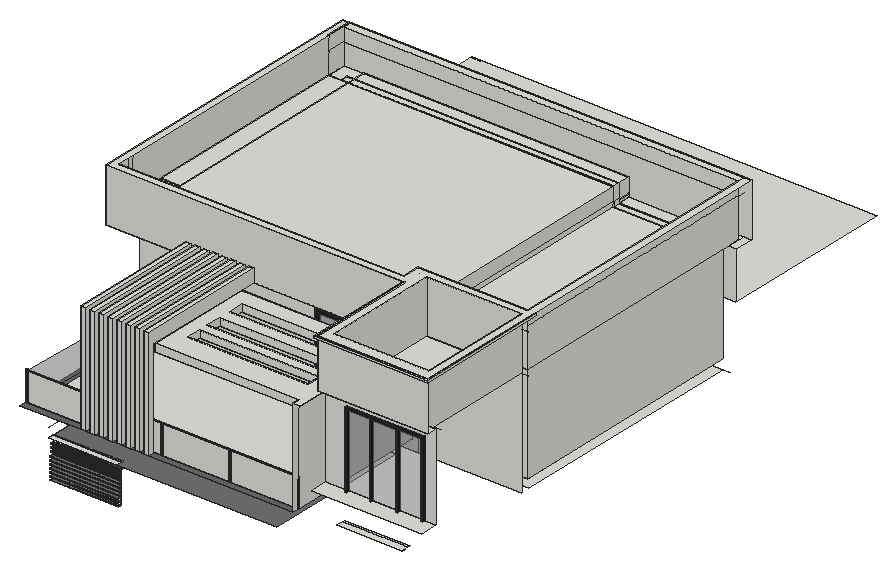
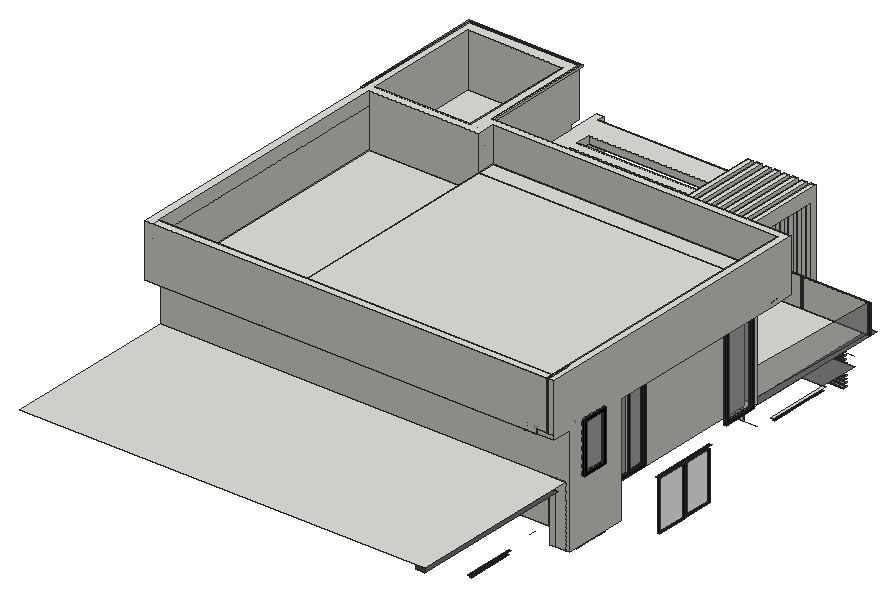
# SketchUp Ruby script. Lengths in inches.
U = 1.inch
M = Sketchup.active_model
def pt(a) = Geom::Point3d.new(a.map { |v| v * U })
def face(e, loops, mat)
  f = e.add_face(loops[0].map { |a| pt(a) })
  loops[1..].each { |l| e.add_face(l.map { |a| pt(a) }).erase! }
  f.material = f.back_material = mat if mat
  f
end
# faces: each face lists its corners as indices into pts; further lists are holes
def faces(e, pts, list, mat = nil) = list.each { |f| face(e, (f[0].is_a?(Array) ? f : [f]).map { |l| l.map { |i| pts[i] } }, mat) }
# xy, xz, yz: faces in a plane at the given z, y or x. An outline is a flat list of corners, or four numbers for a rectangle; further outlines are holes
def ring(l) = l.size == 4 ? [[l[0], l[1]], [l[2], l[1]], [l[2], l[3]], [l[0], l[3]]] : l.each_slice(2).to_a
def flat(e, list, mat, &to3) = list.each { |f| face(e, (f[0].is_a?(Array) ? f : [f]).map { |l| ring(l).map { |u, v| to3.(u, v) } }, mat) }
def xy(e, z, list, mat = nil) = flat(e, list, mat) { |x, y| [x, y, z] }
def xz(e, y, list, mat = nil) = flat(e, list, mat) { |x, z| [x, y, z] }
def yz(e, x, list, mat = nil) = flat(e, list, mat) { |y, z| [x, y, z] }
def lines(e, pts, list) = list.each { |a, b| e.add_line(pt(pts[a]), pt(pts[b])) }
# prism: a flat outline (further loops are holes) pulled along v
def prism(e, loops, v, mat = nil)
  f = face(e, loops, mat); d = Geom::Vector3d.new(v.map { |x| x * U })
  f.pushpull(f.normal.samedirection?(d) ? d.length : -d.length)
end
def box(e, o, s, mat = nil) = prism(e, [[o, [o[0] + s[0], o[1], o[2]], [o[0] + s[0], o[1] + s[1], o[2]], [o[0], o[1] + s[1], o[2]]]], [0, 0, s[2]], mat)
def at(x, y, z, deg = 0) = Geom::Transformation.translation(pt([x, y, z])) * Geom::Transformation.rotation(ORIGIN, Z_AXIS, deg.degrees)
def axes(o, x, y, z) = Geom::Transformation.new([*x, 0, *y, 0, *z, 0, *pt(o).to_a, 1])
def part(name) = M.definitions.add(name)
# library, detail: a bought-in or finely detailed component or shape, given as its bounding box
def library(name, o, s) = part(name).tap { |d| box(d.entities, o, s) }
def detail(e, o, s) = box(e.add_group.entities, o, s)
def put(e, d, t, mat = nil) = e.add_instance(d, t).tap { |i| i.material = mat if mat }
def group(e, t, mat = nil) = e.add_group.tap { |g| g.transformation = t; g.material = mat if mat }.entities
root = M.entities
M.materials.add("[0134_DimGray]").color = [105, 105, 105]
M.materials.add("[0136_Charcoal]").color = [35, 35, 35]
M.materials.add("[0137_Black]").color = [0, 0, 0]
M.materials.add("[Color M05]").color = [114, 114, 114]
M.materials.add("[Color M06]").color = [86, 86, 86]
M.materials.add("[Color M08]").color = [30, 30, 30]
M.materials.add("[Marble Carrara Gold Floor Tile]").color = [225, 223, 217]
M.materials.add("[Translucent Glass Gray]").color = [128, 128, 128]
M.materials["[Translucent Glass Gray]"].alpha = 0.5
c1 = part("Group\#89")
box(c1.entities,[-152.36,0,0],[152.36,1.57,1.57])
c2 = part("Glass+Wall")
g1 = group(c2.entities,at(79.73,0,0))
g2 = group(g1,at(0,0,0))
g3 = group(g2,at(195.28,0,0),"[0136_Charcoal]")
box(g3,[-195.28,0,0],[195.28,1.57,1.57])
put(g2,c1,axes([1.57,0,116.54],[0,0,0.75452],[0,1,0],[-1,0,0]),"[0136_Charcoal]")
put(g2,c1,axes([50,0,116.54],[0,0,0.75452],[0,1,0],[-1,0,0]),"[0136_Charcoal]")
g4 = group(g2,at(195.28,0,115.75),"[0136_Charcoal]")
box(g4,[-195.28,0,0.79],[195.28,1.57,1.57])
put(g2,c1,axes([98.43,0,116.54],[0,0,0.75452],[0,1,0],[-1,0,0]),"[0136_Charcoal]")
put(g2,c1,axes([146.85,0,116.54],[0,0,0.75452],[0,1,0],[-1,0,0]),"[0136_Charcoal]")
put(g2,c1,axes([195.28,0,116.54],[0,0,0.75452],[0,1,0],[-1,0,0]),"[0136_Charcoal]")
g5 = group(g1,at(1.57,0.39,1.57))
box(g5,[0,0,0],[192.125,0.79,114.96])
xy(root,178.66,[[24,306.96,27,342.36],[24,345.3,27,383.64]],"[Color M08]")
xy(root,180.3125,[[61.54,49.95,146.02,53.64]],"[Color M05]")
xy(root,181.39,[[61.54,49.95,146.02,53.64]],"[Color M05]")
xy(root,184.6875,[[61.54,49.95,146.02,53.64]],"[Color M05]")
xy(root,185.77,[[61.54,49.95,146.02,53.64]],"[Color M05]")
xy(root,189.0625,[[61.54,49.95,146.02,53.64]],"[Color M05]")
xy(root,190.14,[[61.54,49.95,146.02,53.64]],"[Color M05]")
xy(root,193.4375,[[61.54,49.95,146.02,53.64]],"[Color M05]")
xy(root,194.52,[[61.54,49.95,146.02,53.64]],"[Color M05]")
xy(root,197.8125,[[61.54,49.95,146.02,53.64]],"[Color M05]")
xy(root,198.89,[[61.54,49.95,146.02,53.64]],"[Color M05]")
xy(root,202.1875,[[61.54,49.95,146.02,53.64]],"[Color M05]")
xy(root,203.27,[[61.54,49.95,146.02,53.64]],"[Color M05]")
xy(root,204,[[161.86,123.29,189.67,123.29,189.67,126.29,233.86,126.29,233.86,129.29,161.86,129.29]])
xy(root,206.5625,[[61.54,49.95,146.02,53.64]],"[Color M05]")
xy(root,207.64,[[61.54,49.95,146.02,53.64]],"[Color M05]")
xy(root,210.9375,[[61.54,50.64,146.02,53.64]],"[Color M05]")
xy(root,212.02,[[61.54,50.64,146.02,53.64]],"[Color M05]")
xy(root,215.3125,[[61.54,50.64,146.02,53.64]],"[Color M05]")
xy(root,216.39,[[61.54,50.64,146.02,53.64]],"[Color M05]")
xy(root,217.37,[[301.27,126.29,303.26,129.29]])
xy(root,217.37,[[280.74,126.29,301.27,129.29],[303.26,126.29,321.8,129.29]],"[Color M08]")
xy(root,218.17,[[24,468.2,27,486.73],[24,489.67,27,511.14]],"[Color M08]")
xy(root,219.6875,[[145.89,50.64,146.02,53.64]])
xy(root,219.6875,[[61.54,50.64,145.89,53.64]],"[Color M05]")
xy(root,220.37,[[277.74,126.29,324.8,129.29]],"[Color M08]")
xy(root,220.77,[[145.89,50.64,146.02,53.64]])
xy(root,220.77,[[61.54,50.64,145.89,53.64],[61.54,53.64,145.89,55.45]],"[Color M05]")
xy(root,221.17,[[24,465.2,27,514.14]])
xy(root,224.0625,[[61.54,53.64,145.89,55.45]],"[Color M05]")
xy(root,225.48,[[24,132.29,27,144.3],[24,146.33,27,160.37],[24,161.62,27,182.61],[24,184.3,27,206.85]],"[Color M08]")
xy(root,228.48,[[61.54,47.14,146.02,53.64],[145.89,53.64,146.02,55.45],[24,129.29,27,209.85],[52.75,129.29,61.54,230.47],[61.54,129.29,342.51,230.47]])
xy(root,228.48,[[146.02,47.14,146.02,55.45,61.54,55.45,61.54,80.27,27,80.27,27,129.29,342.51,129.29,342.51,47.14],[61.54,53.64,145.89,55.45]],"[Color M05]")
xy(root,237.28,[[407.81,74.83,441.65,77.83],[445.14,74.83,475.49,77.83]],"[Color M06]")
xy(root,238.0625,[[3,469.72,27,548.83]])
xy(root,238.72,[[24,306.96,27,342.36],[24,345.3,27,383.64]],"[Color M08]")
xy(root,240,[[43.75,80.27,61.54,230.47],[52.75,230.47,61.54,242.39],[61.54,230.47,371,242.39],[371,242.39,496.75,539.83]])
xy(root,241.72,[[24,303.96,27,386.64]],"[Color M08]")
xy(root,243.28,[[401.81,65.83,481.49,74.83],[401.81,74.83,481.49,77.83]])
xy(root,252,[[36,239.47,496.75,539.83]])
xy(root,252,[[27,47.14,101.33,47.14,101.33,54.84,107.83,54.84,107.83,47.14,112.39,47.14,112.39,54.62,118.89,54.62,118.89,47.14,123.45,47.14,123.45,53.91,129.95,53.91,129.95,47.14,134.51,47.14,134.51,53.23,141.01,53.23,141.01,47.14,145.58,47.14,145.58,53.64,152.08,53.64,152.08,47.14,156.64,47.14,156.64,53.64,163.14,53.64,163.14,47.14,167.7,47.14,167.7,54.2,174.2,54.2,174.2,47.14,178.76,47.14,178.76,53.64,185.26,53.64,185.26,47.14,362,47.14,362,56.14,36,56.14,36,230.47,27,230.47]],"[0134_DimGray]")
xy(root,252,[[36,56.14,362,230.47]],"[Marble Carrara Gold Floor Tile]")
xy(root,252.8125,[[24,239.47,27,281.29]])
xy(root,255.8125,[[24,242.47,27,278.29]],"[Color M08]")
xy(root,263.61,[[24,405.68,27,454.62]])
xy(root,263.93,[[16.75,624.57,19.75,681.82]],"[Color M08]")
xy(root,266.61,[[24,408.68,27,430.15],[24,432.86,27,451.62]],"[Color M08]")
xy(root,266.93,[[16.75,621.57,19.75,684.82]],"[Color M08]")
xy(root,270.8125,[[371,65.83,505.75,65.83,505.75,86.83,492.95,86.83,492.95,83.83,489.95,83.83,489.95,86.83,462.06,86.83,462.06,83.83,459.625,83.83,459.625,86.83,429.3,86.83,429.3,83.83,426.98,83.83,426.98,86.83,399.39,86.83,399.39,83.83,396.39,83.83,396.39,86.83,371,86.83],[396.39,83.83,399.39,86.83],[426.98,83.83,429.3,86.83],[459.625,83.83,462.06,86.83],[489.95,83.83,492.95,86.83]])
xy(root,277.23,[[245.29,227.47,307.6,230.47]])
xy(root,280.23,[[248.29,227.47,276.44,230.47],[277.62,227.47,304.6,230.47]],"[Color M08]")
xy(root,308.3,[[7.75,560.23,19.75,764.77]],"[Color M06]")
xy(root,313.57,[[0,496.85,3,529.73]],"[0137_Black]")
xy(root,313.6875,[[7.75,548.83,505.75,764.77]])
xy(root,316.57,[[0,499.85,3,526.73]],"[0137_Black]")
xy(root,352.92,[[248.29,227.47,276.44,230.47],[277.62,227.47,304.6,230.47]],"[Color M08]")
xy(root,355.92,[[245.29,227.47,307.6,230.47]],"[Color M08]")
xy(root,359.86,[[24,408.68,27,430.15],[24,432.86,27,451.62]],"[Color M08]")
xy(root,361.3125,[[399.39,83.83,426.98,86.83],[429.3,83.83,459.625,86.83],[462.06,83.83,489.95,86.83]],"[Color M08]")
xy(root,362.86,[[24,405.68,27,454.62]],"[Color M08]")
xy(root,363.09,[[[185.26,56.14,362,189.36],[202.36,85.48,349.98,104.1],[202.36,115.35,349.98,133.98],[202.36,149.29,349.98,167.91]]])
xy(root,364.3125,[[396.39,83.83,492.95,86.83]],"[Color M08]")
xy(root,369,[[24,242.47,27,278.29]],"[Color M08]")
xy(root,372,[[[362,47.14,371,47.14,371,208.85,362,208.85,362,189.36,185.26,189.36,185.26,56.14,362,56.14],[202.36,149.29,349.98,167.91],[202.36,115.35,349.98,133.98],[202.36,85.48,349.98,104.1]],[134.51,53.23,141.01,208.85],[145.58,53.64,152.08,208.85],[156.64,53.64,163.14,208.85],[178.76,53.64,185.26,208.85],
  [123.45,53.91,129.95,208.85],[167.7,54.2,174.2,208.85],[112.39,54.62,118.89,208.85],[101.33,54.84,107.83,208.85],[380,87.77,496.75,230.47],
  [371,95.83,380,230.47],[3,208.85,3,239.47,27,239.47,27,230.47,362,230.47,362,208.85],[362,208.85,371,230.47],[27,230.47,36,239.47],[36,230.47,362,239.47],
  [3,239.47,3,469.72,27,469.72,27,281.29,24,281.29,24,239.47],[24,239.47,27,239.54],[27,239.47,36,239.54],[36,239.47,362,239.54],[362,239.47,496.75,539.83],
  [24,239.54,27,281.29],[27,239.54,36,281.29],[36,239.54,362,539.83],[27,281.29,36,539.83],[23.0625,539.83,23.5,540.72],
  [23.5,539.83,24,540.72],[24,539.83,27,540.72],[27,539.83,36,540.72],[36,539.83,362,540.72],[362,539.83,496.75,548.83],
  [23.0625,540.72,23.5,548.83],[23.5,540.72,24,548.83],[24,540.72,27,548.83],[27,540.72,36,548.83],[36,540.72,362,548.83],
  [3,548.83,3,572.85,24,572.85,24,572.83,23.5,572.83,23.5,548.83],[23.5,548.83,24,572.83],[24,548.83,27,572.83],[27,548.83,36,572.83],[36,548.83,362,572.83],
  [362,548.83,496.75,572.83],[496.75,548.83,505.75,572.83],[24,572.83,27,572.85],[27,572.83,36,572.85],[36,572.83,362,572.85]])
xy(root,372.625,[[362,548.83,496.75,563.83]])
xy(root,373.26,[[0,499.85,3,526.73]],"[0137_Black]")
xy(root,374.25,[[36,548.83,362,563.83]])
xy(root,376.26,[[0,496.85,3,529.73]],"[0137_Black]")
xy(root,377.09,[[371,74.83,505.75,86.83]])
xy(root,377.125,[[12,216.41,36,281.29],[12,539.83,23.5,563.83],[23.5,539.83,27,563.83],[27,539.83,36,563.83]])
xy(root,377.4375,[[36,230.47,36.75,239.47],[36,230.47,36.75,239.47],[10.125,540.72,12,572.83],[12,563.83,23.5,572.83]])
xy(root,387.625,[[101.33,47.14,107.83,208.85],[112.39,47.14,118.89,208.85],[123.45,47.14,129.95,208.85],[134.51,47.14,141.01,208.85],[145.58,47.14,152.08,208.85],
  [156.64,47.14,163.14,208.85],[167.7,47.14,174.2,208.85],[178.76,47.14,185.26,208.85]])
xy(root,394.3125,[[12,216.41,36,281.29],[36,217.85,362,239.54],[36,239.54,362,539.83],[12,281.29,36,539.83],[12,539.83,36,539.83,36,540.72,27,540.72,27,548.83,36,548.83,36,563.83,12,563.83],
  [27,540.72,36,548.83],[36,540.72,362,548.83],[36,548.83,362,563.83]])
xy(root,435.13,[[368.375,71.83,368.375,208.85,371,208.85,371,74.83,505.75,74.83,505.75,238.52,508.125,238.52,508.125,71.83]])
xy(root,437.4375,[[368.375,71.83,508.125,71.83,508.125,238.52,505.75,238.52,505.75,74.83,371,74.83,371,208.85,368.375,208.85],[[371,74.83,505.75,74.83,505.75,572.83,496.75,572.83,496.75,239.47,362,239.47,362,217.85,12,217.85,12,540.72,10.125,540.72,10.125,572.83,12,572.83,12,572.85,3,572.85,3,208.85,371,208.85],[380,87.77,496.75,230.47]],[10.125,540.72,12,572.83],[12,563.83,496.75,572.83]])
xz(root,47.14,[[101.33,252,107.83,387.625],[112.39,252,118.89,387.625],[123.45,252,129.95,387.625],[134.51,252,141.01,387.625],[145.58,252,152.08,387.625],
  [156.64,252,163.14,387.625],[167.7,252,174.2,387.625],[178.76,252,185.26,387.625]])
xz(root,49.95,[[61.54,180.3125,146.02,181.39],[61.54,184.6875,146.02,185.77],[61.54,189.0625,146.02,190.14],[61.54,193.4375,146.02,194.52],[61.54,197.8125,146.02,198.89],
  [61.54,202.1875,146.02,203.27],[61.54,206.5625,146.02,207.64]],"[Color M05]")
xz(root,50.64,[[145.89,219.6875,146.02,220.77]])
xz(root,50.64,[[61.54,210.9375,146.02,212.02],[61.54,215.3125,146.02,216.39],[61.54,219.6875,145.89,220.77]],"[Color M05]")
xz(root,53.23,[[134.51,252,141.01,372]])
xz(root,53.64,[[61.54,180.3125,145.89,181.39],[145.89,180.3125,146.02,181.39],[145.89,181.39,146.02,184.6875],[61.54,184.6875,145.89,185.77],[145.89,184.6875,146.02,185.77],
  [145.89,185.77,146.02,189.0625],[61.54,189.0625,145.89,190.14],[145.89,189.0625,146.02,190.14],[145.89,190.14,146.02,193.4375],[61.54,193.4375,145.89,194.52],
  [145.89,193.4375,146.02,194.52],[145.89,194.52,146.02,197.8125],[61.54,197.8125,145.89,198.89],[145.89,197.8125,146.02,198.89],[145.89,198.89,146.02,202.1875],
  [61.54,202.1875,145.89,203.27],[145.89,202.1875,146.02,203.27],[145.89,203.27,146.02,206.5625],[61.54,206.5625,145.89,207.64],[145.89,206.5625,146.02,207.64],
  [145.89,207.64,146.02,210.9375],[61.54,210.9375,145.89,212.02],[145.89,210.9375,146.02,212.02],[145.89,212.02,146.02,215.3125],[61.54,215.3125,145.89,216.39],
  [145.89,215.3125,146.02,216.39],[145.89,216.39,146.02,219.6875],[61.54,219.6875,146.02,220.77],[145.89,220.77,146.02,224.0625],[145.89,224.0625,146.02,225.14],
  [145.89,225.14,146.02,228.4375],[61.54,228.4375,145.89,228.48],[145.89,228.4375,146.02,228.48],[145.58,252,152.08,372],[156.64,252,163.14,372],
  [178.76,252,185.26,372]])
xz(root,53.64,[[61.54,224.0625,145.89,225.14]],"[Color M05]")
xz(root,53.91,[[123.45,252,129.95,372]])
xz(root,54.2,[[167.7,252,174.2,372]])
xz(root,54.62,[[112.39,252,118.89,372]])
xz(root,54.84,[[101.33,252,107.83,372]])
xz(root,55.45,[[145.89,220.77,146.02,224.0625],[145.89,224.0625,146.02,228.48]])
xz(root,56.14,[[185.26,363.09,362,372]])
xz(root,71.83,[[368.375,435.13,508.125,437.4375]])
xz(root,74.83,[[371,377.09,505.75,435.13],[371,435.13,505.75,437.4375]])
xz(root,80.27,[[27,228.4375,61.54,228.48]])
xz(root,83.83,[[396.39,270.8125,399.39,270.8125,399.39,361.3125,426.98,361.3125,426.98,270.8125,429.3,270.8125,429.3,361.3125,459.625,361.3125,459.625,270.8125,462.06,270.8125,462.06,361.3125,489.95,361.3125,489.95,270.8125,492.95,270.8125,492.95,364.3125,396.39,364.3125]],"[Color M08]")
xz(root,85.48,[[202.36,363.09,349.98,372]])
xz(root,86.83,[[371,270.8125,396.39,270.8125,396.39,364.3125,492.95,364.3125,492.95,270.8125,505.75,270.8125,505.75,377.09,371,377.09],[396.39,270.8125,396.39,364.3125,492.95,364.3125,492.95,270.8125,489.95,270.8125,489.95,361.3125,462.06,361.3125,462.06,270.8125,459.625,270.8125,459.625,361.3125,429.3,361.3125,429.3,270.8125,426.98,270.8125,426.98,361.3125,399.39,361.3125,399.39,270.8125]])
xz(root,86.83,[[399.39,270.8125,426.98,361.3125],[429.3,270.8125,459.625,361.3125],[462.06,270.8125,489.95,361.3125]],"[Translucent Glass Gray]")
xz(root,87.77,[[380,372,496.75,437.4375]])
xz(root,104.1,[[202.36,363.09,349.98,372]])
xz(root,115.35,[[202.36,363.09,349.98,372]])
xz(root,133.98,[[202.36,363.09,349.98,372]])
xz(root,149.29,[[202.36,363.09,349.98,372]])
xz(root,167.91,[[202.36,363.09,349.98,372]])
xz(root,189.36,[[185.26,363.09,362,372]])
xz(root,208.85,[[3,372,101.33,372,101.33,387.625,107.83,387.625,107.83,372,112.39,372,112.39,387.625,118.89,387.625,118.89,372,123.45,372,123.45,387.625,129.95,387.625,129.95,372,134.51,372,134.51,387.625,141.01,387.625,141.01,372,145.58,372,145.58,387.625,152.08,387.625,152.08,372,156.64,372,156.64,387.625,163.14,387.625,163.14,372,167.7,372,167.7,387.625,174.2,387.625,174.2,372,178.76,372,178.76,387.625,185.26,387.625,185.26,372,371,372,371,435.13,368.375,435.13,368.375,437.4375,3,437.4375],[101.33,372,107.83,387.625],[112.39,372,118.89,387.625],[123.45,372,129.95,387.625],[134.51,372,141.01,387.625],
  [145.58,372,152.08,387.625],[156.64,372,163.14,387.625],[167.7,372,174.2,387.625],[178.76,372,185.26,387.625]])
xz(root,216.41,[[12,377.125,36,394.3125]])
xz(root,217.85,[[12,377.4375,12,437.4375,362,437.4375,362,394.3125,36,394.3125,36,377.4375],[36,377.4375,362,394.3125]])
xz(root,227.47,[[[245.29,277.23,307.6,355.92],[248.29,280.23,276.44,352.92],[277.62,280.23,304.6,352.92]]],"[Color M08]")
xz(root,230.47,[[43.75,228.48,44.27,240],[44.27,228.48,52.75,240],[52.75,228.48,61.54,240],[44.27,240,371,240,371,372,362,372,362,252,44.27,252],[371,240,496.75,372],
  [[27,252,362,372],[245.29,277.23,307.6,355.92]],[371,372,380,420.6875],[380,372,496.75,437.4375]])
xz(root,230.47,[[248.29,280.23,276.44,352.92],[277.62,280.23,304.6,352.92]],"[Translucent Glass Gray]")
xz(root,238.52,[[505.75,435.13,508.125,437.4375]])
xz(root,239.47,[[36,252,496.75,372],[362,372,496.75,437.4375],[36,377.125,36.75,377.4375]])
xz(root,239.47,[[24,252.8125,27,372]],"[Color M08]")
xz(root,239.54,[[36,372,362,394.3125]])
xz(root,242.47,[[24,255.8125,27,369]],"[Color M08]")
xz(root,278.29,[[24,255.8125,27,369]],"[Color M08]")
xz(root,281.29,[[12,377.125,36,394.3125]])
xz(root,281.29,[[24,252.8125,27,372]],"[Color M08]")
xz(root,306.96,[[24,178.66,27,238.72]],"[Color M08]")
xz(root,342.36,[[24,178.66,27,238.72]],"[Color M08]")
xz(root,345.3,[[24,178.66,27,238.72]],"[Color M08]")
xz(root,383.64,[[24,178.66,27,238.72]],"[Color M08]")
xz(root,405.68,[[24,263.61,27,362.86]],"[Color M08]")
xz(root,408.68,[[24,266.61,27,359.86]],"[Color M08]")
xz(root,430.15,[[24,266.61,27,359.86]],"[Color M08]")
xz(root,432.86,[[24,266.61,27,359.86]])
xz(root,451.62,[[24,266.61,27,359.86]],"[Color M08]")
xz(root,454.62,[[24,263.61,27,362.86]])
xz(root,469.72,[[3,238.0625,27,372]])
xz(root,496.85,[[0,313.57,3,376.26]],"[0137_Black]")
xz(root,499.85,[[0,316.57,3,373.26]],"[0137_Black]")
xz(root,526.73,[[0,316.57,3,373.26]],"[0137_Black]")
xz(root,529.73,[[0,313.57,3,376.26]],"[0137_Black]")
xz(root,539.83,[[36,252,496.75,372],[23.5,372,27,377.125],[27,372,36,377.125],[36,372,362,394.3125],[12,377.125,36,394.3125]])
xz(root,540.72,[[27,372,36,394.3125],[36,372,362,394.3125],[10.125,377.4375,12,379.75],[10.125,379.75,12,420.6875],[10.125,420.6875,12,437.4375]])
xz(root,548.83,[[3,238.0625,3,372,505.75,372,505.75,313.6875,7.75,313.6875,7.75,238.0625],[7.75,238.0625,19.75,313.6875],[19.75,238.0625,27,313.6875],[27,372,36,379.75],[36,372,362,374.25],
  [362,372,496.75,372.625],[36,374.25,362,394.3125],[27,379.75,36,394.3125]])
xz(root,563.83,[[362,372.625,496.75,372.625,496.75,420.6875,12,420.6875,12,394.3125,362,394.3125],[36,374.25,362,394.3125],[12,377.125,23.5,377.4375],[23.5,377.125,27,377.4375],[12,420.6875,496.75,437.4375]])
xz(root,572.83,[[23.5,372,23.5,377.4375,10.125,377.4375,10.125,437.4375,505.75,437.4375,505.75,372]])
xz(root,572.85,[[3,372,24,377.4375],[3,377.4375,12,437.4375]])
xz(root,764.77,[[7.75,308.3,19.75,313.6875]],"[Color M06]")
yz(root,0,[[[496.85,313.57,529.73,376.26],[499.85,316.57,526.73,373.26]]],"[0137_Black]")
yz(root,3,[[[469.72,238.0625,469.72,372,239.47,372,239.47,377.125,239.54,377.125,239.54,377.4375,230.47,377.4375,230.47,377.125,239.47,377.125,239.47,372,208.85,372,208.85,437.4375,572.85,437.4375,572.85,372,548.83,372,548.83,238.0625],[496.85,313.57,529.73,376.26]],[[496.85,313.57,529.73,376.26],[499.85,316.57,526.73,373.26]],[230.47,377.125,239.54,377.4375]])
yz(root,3,[[499.85,316.57,526.73,373.26]],"[Translucent Glass Gray]")
yz(root,10.125,[[540.72,377.4375,572.83,420.6875],[540.72,420.6875,572.83,437.4375]])
yz(root,12,[[216.41,377.125,281.29,377.4375],[539.83,377.125,563.83,377.4375],[216.41,377.4375,217.85,394.3125],[217.85,377.4375,230.47,394.3125],[230.47,377.4375,239.54,394.3125],
  [239.54,377.4375,281.29,394.3125],[281.29,377.4375,539.83,394.3125],[539.83,377.4375,540.72,394.3125],[540.72,377.4375,563.83,394.3125],[563.83,377.4375,572.85,437.4375],
  [217.85,394.3125,230.47,437.4375],[230.47,394.3125,239.54,437.4375],[239.54,394.3125,540.72,437.4375],[540.72,394.3125,563.83,420.6875],[540.72,420.6875,563.83,437.4375]])
yz(root,23.5,[[539.83,372,539.83,377.125,563.83,377.125,563.83,377.4375,572.83,377.4375,572.83,372]])
yz(root,24,[[[239.47,252.8125,281.29,372],[242.47,255.8125,278.29,369]],[[405.68,263.61,454.62,362.86],[408.68,266.61,430.15,359.86],[432.86,266.61,451.62,359.86]]],"[Color M08]")
yz(root,27,[[469.72,238.0625,539.83,372],[[239.47,252.8125,281.29,372],[242.47,255.8125,278.29,369]],[539.83,372,540.72,377.125],[540.72,372,548.83,377.125],[540.72,377.125,548.83,394.3125]])
yz(root,27,[[306.96,178.66,342.36,238.72],[345.3,178.66,383.64,238.72],[242.47,255.8125,278.29,369],[408.68,266.61,430.15,359.86],[432.86,266.61,451.62,359.86]],"[Translucent Glass Gray]")
yz(root,36,[[239.47,252,539.83,372],[239.47,372,239.54,377.125],[239.54,372,281.29,377.125],[281.29,372,539.83,394.3125],[540.72,372,548.83,377.125],
  [548.83,372,563.83,374.25],[548.83,374.25,563.83,377.125],[216.41,377.125,217.85,394.3125],[217.85,377.125,239.54,394.3125],[239.54,377.125,281.29,394.3125],
  [539.83,377.125,540.72,394.3125],[540.72,377.125,548.83,394.3125],[548.83,377.125,563.83,379.75],[548.83,379.75,563.83,394.3125]])
yz(root,61.54,[[49.95,180.3125,53.64,181.39],[49.95,184.6875,53.64,185.77],[49.95,189.0625,53.64,190.14],[49.95,193.4375,53.64,194.52],[49.95,197.8125,53.64,198.89],
  [49.95,202.1875,53.64,203.27],[49.95,206.5625,53.64,207.64],[50.64,210.9375,53.64,212.02],[50.64,215.3125,53.64,216.39],[53.64,224.0625,55.45,228.4375],
  [47.14,228.4375,53.64,228.48],[53.64,228.4375,55.45,228.48],[55.45,228.4375,80.27,228.48]])
yz(root,101.33,[[47.14,252,47.14,387.625,208.85,387.625,208.85,372,54.84,372,54.84,252]])
yz(root,107.83,[[47.14,252,54.84,252,54.84,372,208.85,372,208.85,387.625,47.14,387.625]])
yz(root,112.39,[[47.14,252,47.14,387.625,208.85,387.625,208.85,372,54.62,372,54.62,252]])
yz(root,118.89,[[47.14,252,54.62,252,54.62,372,208.85,372,208.85,387.625,47.14,387.625]])
yz(root,123.45,[[47.14,252,47.14,387.625,208.85,387.625,208.85,372,53.91,372,53.91,252]])
yz(root,129.95,[[47.14,252,53.91,252,53.91,372,208.85,372,208.85,387.625,47.14,387.625]])
yz(root,134.51,[[47.14,252,47.14,387.625,208.85,387.625,208.85,372,53.23,372,53.23,252]])
yz(root,141.01,[[47.14,252,53.23,252,53.23,372,208.85,372,208.85,387.625,47.14,387.625]])
yz(root,145.58,[[47.14,252,47.14,387.625,208.85,387.625,208.85,372,53.64,372,53.64,252]])
yz(root,145.89,[[53.64,220.77,55.45,224.0625],[53.64,224.0625,55.45,228.48]])
yz(root,146.02,[[49.95,180.3125,53.64,181.39],[49.95,184.6875,53.64,185.77],[49.95,189.0625,53.64,190.14],[49.95,193.4375,53.64,194.52],[49.95,197.8125,53.64,198.89],
  [49.95,202.1875,53.64,203.27],[49.95,206.5625,53.64,207.64],[50.64,210.9375,53.64,212.02],[50.64,215.3125,53.64,216.39],[50.64,219.6875,53.64,220.77]],"[Color M05]")
yz(root,152.08,[[47.14,252,53.64,252,53.64,372,208.85,372,208.85,387.625,47.14,387.625]])
yz(root,156.64,[[47.14,252,47.14,387.625,208.85,387.625,208.85,372,53.64,372,53.64,252]])
yz(root,163.14,[[47.14,252,53.64,252,53.64,372,208.85,372,208.85,387.625,47.14,387.625]])
yz(root,167.7,[[47.14,252,47.14,387.625,208.85,387.625,208.85,372,54.2,372,54.2,252]])
yz(root,174.2,[[47.14,252,54.2,252,54.2,372,208.85,372,208.85,387.625,47.14,387.625]])
yz(root,178.76,[[47.14,252,47.14,387.625,208.85,387.625,208.85,372,53.64,372,53.64,252]])
yz(root,185.26,[[47.14,252,53.64,252,53.64,372,208.85,372,208.85,387.625,47.14,387.625],[56.14,363.09,189.36,372]])
yz(root,202.36,[[85.48,363.09,104.1,372],[115.35,363.09,133.98,372],[149.29,363.09,167.91,372]])
yz(root,245.29,[[227.47,277.23,230.47,355.92]],"[Color M08]")
yz(root,248.29,[[227.47,280.23,230.47,352.92]],"[Color M08]")
yz(root,276.44,[[227.47,280.23,230.47,352.92]],"[Color M08]")
yz(root,277.62,[[227.47,280.23,230.47,352.92]],"[Color M08]")
yz(root,304.6,[[227.47,280.23,230.47,352.92]],"[Color M08]")
yz(root,307.6,[[227.47,277.23,230.47,355.92]],"[Color M08]")
yz(root,349.98,[[85.48,363.09,104.1,372],[115.35,363.09,133.98,372],[149.29,363.09,167.91,372]])
yz(root,362,[[47.14,252,56.14,372],[56.14,252,56.14,363.09,189.36,363.09,189.36,372,230.47,372,230.47,252],[217.85,372,230.47,377.4375],[230.47,372,239.47,377.4375],[239.47,372,239.54,377.4375],
  [239.54,372,539.83,377.4375],[539.83,372,540.72,377.4375],[540.72,372,548.83,377.4375],[548.83,372,563.83,372.625],[548.83,372.625,563.83,374.25],
  [548.83,374.25,563.83,377.4375],[217.85,377.4375,230.47,394.3125],[230.47,377.4375,239.47,394.3125],[239.47,377.4375,239.54,394.3125],[239.54,377.4375,539.83,394.3125],
  [540.72,377.4375,548.83,394.3125],[548.83,377.4375,563.83,394.3125],[217.85,394.3125,239.47,437.4375]])
yz(root,368.375,[[71.83,435.13,208.85,437.4375]])
yz(root,371,[[86.83,372,86.83,377.09,74.83,377.09,74.83,435.13,208.85,435.13,208.85,372],[74.83,435.13,208.85,437.4375]])
yz(root,380,[[87.77,372,230.47,437.4375]])
yz(root,396.39,[[83.83,270.8125,86.83,364.3125]],"[Color M08]")
yz(root,399.39,[[83.83,270.8125,86.83,361.3125]],"[Color M08]")
yz(root,426.98,[[83.83,270.8125,86.83,361.3125]],"[Color M08]")
yz(root,429.3,[[83.83,270.8125,86.83,361.3125]],"[Color M08]")
yz(root,459.625,[[83.83,270.8125,86.83,361.3125]],"[Color M08]")
yz(root,462.06,[[83.83,270.8125,86.83,361.3125]],"[Color M08]")
yz(root,489.95,[[83.83,270.8125,86.83,361.3125]],"[Color M08]")
yz(root,492.95,[[83.83,270.8125,86.83,364.3125]],"[Color M08]")
yz(root,496.75,[[239.47,252,539.83,372],[87.77,372,230.47,437.4375],[239.47,372,239.47,420.6875,563.83,420.6875,563.83,372.625,548.83,372.625,548.83,372],[548.83,372,563.83,372.625],[239.47,420.6875,563.83,437.4375]])
yz(root,505.75,[[74.83,435.13,238.52,437.4375]])
yz(root,508.125,[[71.83,435.13,238.52,437.4375]])
p = [[36,230.47,252],[29.7,56.14,252],[29.7,56.14,287.64],[36,230.47,287.64],[61.54,47.14,240],[61.54,80.27,240],
  [43.75,80.27,240],[27,80.27,240],[43.75,80.27,228.48],[43.75,230.47,228.48],[27,230.47,228.48],[371,539.83,240],
  [371,548.83,240],[52.75,539.83,240],[52.75,548.83,240],[496.75,539.83,240],[505.75,539.83,240],[362,230.47,252],
  [362,239.47,252],[371,230.47,420.6875],[362,230.47,420.6875],[505.75,230.47,420.6875],[496.75,230.47,420.6875],[36.75,230.47,377.125],
  [36.75,230.47,377.4375],[36,230.47,377.125],[353,239.47,377.4375],[353,239.54,377.4375],[496.75,563.83,420.6875],[496.75,572.83,420.6875],
  [36,563.83,377.125],[36,572.83,377.125],[27,539.83,377.4375],[27,539.83,377.125],[27,563.83,377.4375],[27,572.85,377.4375],
  [24,540.72,372],[24,540.72,379.75],[12,540.72,379.75],[24,572.85,379.75],[10.125,540.72,379.75],[3,540.72,379.75],
  [12,281.29,372],[12,281.29,377.125],[12,539.83,372],[12,539.83,377.125],[3,539.83,377.125],[36,217.85,372],
  [36,217.85,377.125],[36,563.83,379.75],[36,572.83,379.75],[362,563.83,377.4375],[362,572.85,377.4375],[27,548.83,379.75],
  [27,572.83,379.75],[362,217.85,420.6875],[362,208.85,420.6875],[362,217.85,394.3125],[362,208.85,394.3125],[362,217.85,377.4375],
  [362,208.85,377.4375],[496.75,230.47,372],[505.75,230.47,372],[496.75,95.83,372],[505.75,95.83,372],[371,230.47,437.4375],
  [496.75,86.83,372],[496.75,87.77,372]]
faces(root,p,[[0,1,2,3]],"[Translucent Glass Gray]")
lines(root,p,[[4,5],[6,7],[6,8],[9,10],[11,12],[13,14],[15,16],[17,18],[19,20],[21,22],[23,24],[23,25],
  [26,27],[28,29],[30,31],[32,33],[34,35],[36,37],[37,38],[37,39],[40,41],[42,43],[44,45],[45,46],
  [47,48],[49,50],[51,52],[53,54],[55,56],[57,58],[59,60],[61,62],[63,64],[19,65],[66,67]])
put(root,c2,axes([-109.77,55.65,251.51],[1.71552,0,0],[0,0.31,0],[0,0,0.31]))
